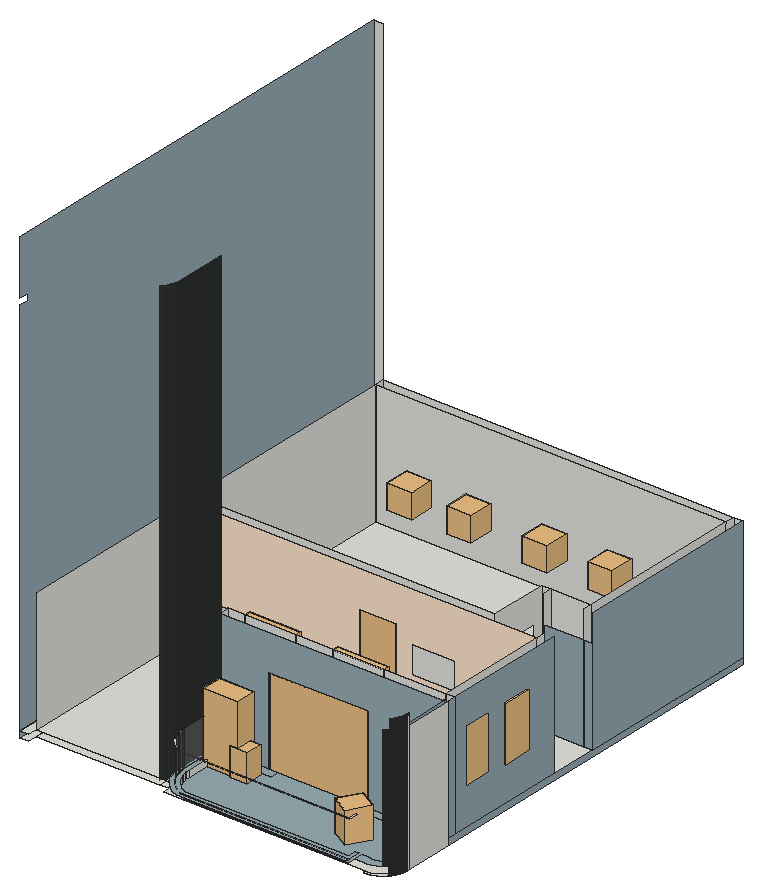
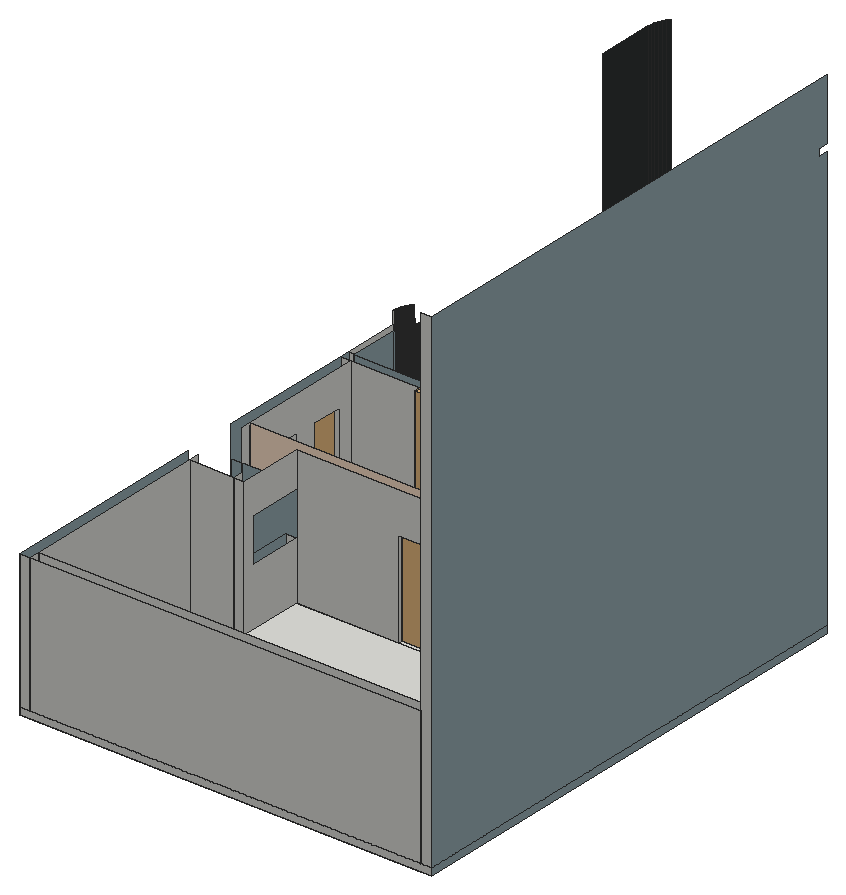
# SketchUp Ruby script. Lengths in inches.
U = 1.inch
M = Sketchup.active_model
def pt(a) = Geom::Point3d.new(a.map { |v| v * U })
def face(e, loops, mat)
  f = e.add_face(loops[0].map { |a| pt(a) })
  loops[1..].each { |l| e.add_face(l.map { |a| pt(a) }).erase! }
  f.material = f.back_material = mat if mat
  f
end
# faces: each face lists its corners as indices into pts; further lists are holes
def faces(e, pts, list, mat = nil) = list.each { |f| face(e, (f[0].is_a?(Array) ? f : [f]).map { |l| l.map { |i| pts[i] } }, mat) }
# xy, xz, yz: faces in a plane at the given z, y or x. An outline is a flat list of corners, or four numbers for a rectangle; further outlines are holes
def ring(l) = l.size == 4 ? [[l[0], l[1]], [l[2], l[1]], [l[2], l[3]], [l[0], l[3]]] : l.each_slice(2).to_a
def flat(e, list, mat, &to3) = list.each { |f| face(e, (f[0].is_a?(Array) ? f : [f]).map { |l| ring(l).map { |u, v| to3.(u, v) } }, mat) }
def xy(e, z, list, mat = nil) = flat(e, list, mat) { |x, y| [x, y, z] }
def xz(e, y, list, mat = nil) = flat(e, list, mat) { |x, z| [x, y, z] }
def yz(e, x, list, mat = nil) = flat(e, list, mat) { |y, z| [x, y, z] }
def lines(e, pts, list) = list.each { |a, b| e.add_line(pt(pts[a]), pt(pts[b])) }
# prism: a flat outline (further loops are holes) pulled along v
def prism(e, loops, v, mat = nil)
  f = face(e, loops, mat); d = Geom::Vector3d.new(v.map { |x| x * U })
  f.pushpull(f.normal.samedirection?(d) ? d.length : -d.length)
end
def box(e, o, s, mat = nil) = prism(e, [[o, [o[0] + s[0], o[1], o[2]], [o[0] + s[0], o[1] + s[1], o[2]], [o[0], o[1] + s[1], o[2]]]], [0, 0, s[2]], mat)
def at(x, y, z, deg = 0) = Geom::Transformation.translation(pt([x, y, z])) * Geom::Transformation.rotation(ORIGIN, Z_AXIS, deg.degrees)
def axes(o, x, y, z) = Geom::Transformation.new([*x, 0, *y, 0, *z, 0, *pt(o).to_a, 1])
def part(name) = M.definitions.add(name)
# library, detail: a bought-in or finely detailed component or shape, given as its bounding box
def library(name, o, s) = part(name).tap { |d| box(d.entities, o, s) }
def detail(e, o, s) = box(e.add_group.entities, o, s)
def put(e, d, t, mat = nil) = e.add_instance(d, t).tap { |i| i.material = mat if mat }
def group(e, t, mat = nil) = e.add_group.tap { |g| g.transformation = t; g.material = mat if mat }.entities
root = M.entities
M.materials.add("Generic").color = [150, 171, 178]
M.materials.add("Generic\#1").color = [47, 50, 50]
M.materials.add("Glass Thin Clear 001").color = [252, 250, 250]
M.materials["Glass Thin Clear 001"].alpha = 0.1
M.materials.add("[Color C01]").color = [255, 229, 204]
c1 = library("Chair 288 019",[-10.59,-11.4,0],[21.2,22.8,30.25])
c2 = library("Potted Plant 50-24",[-2.18,-2.1,0],[4.36,4.2,6.7])
c3 = library("Plant 260 020",[-18.86,-7.03,0.01],[33.61,20.04,67.26])
c4 = library("Window 46-47",[-61.02,-2.17,0],[122.04,4.34,74.02])
c5 = library("Curtains 003",[-24.98,-2.79,0.01],[49.96,5.58,117.31])
c6 = library("Window 46-05",[-17.86,-2.78,0],[35.72,4.26,58.96])
c7 = library("Door 243 053",[-21.6,-2.79,-0.07],[43.2,5.58,82.64])
c8 = library("Omni Light",[-12,-12,-12],[24,24,24])
xy(root,120,[[337.222,41.748,337.222,42.0625,337.846,42.071,338.474,42.095,339.101,42.136,339.726,42.194,340.35,42.268,340.972,42.358,341.591,42.464,342.207,42.587,342.82,42.726,343.429,42.88,344.034,43.051,344.634,43.237,345.229,43.439,345.818,43.657,346.402,43.889,346.979,44.137,347.55,44.4,348.113,44.678,348.669,44.971,349.218,45.278,349.758,45.599,350.289,45.934,350.811,46.283,351.324,46.646,351.828,47.022,352.321,47.411,352.804,47.813,353.277,48.227,353.738,48.654,354.188,49.092,354.627,49.542,355.053,50.003,355.467,50.476,355.869,50.959,356.258,51.452,356.634,51.956,356.997,52.469,357.346,52.991,357.681,53.523,358.002,54.0625,358.309,54.611,358.602,55.167,358.88,55.73,359.143,56.301,359.391,56.878,359.624,57.462,359.841,58.051,360.043,58.646,360.229,59.246,360.4,59.851,360.554,60.46,360.693,61.073,360.816,61.689,360.922,62.308,361.012,62.93,361.086,63.554,361.144,64.179,361.185,64.806,361.209,65.434,361.218,66.0625,361.532,66.058,361.523,65.426,361.498,64.79,361.457,64.155,361.399,63.521,361.324,62.889,361.232,62.259,361.125,61.632,361,61.007,360.86,60.386,360.703,59.77,360.531,59.157,360.342,58.549,360.137,57.946,359.917,57.349,359.681,56.758,359.43,56.173,359.163,55.595,358.882,55.024,358.585,54.461,358.274,53.905,357.949,53.358,357.609,52.82,357.256,52.291,356.888,51.771,356.507,51.261,356.113,50.761,355.706,50.272,355.287,49.793,354.854,49.326,354.41,48.87,353.954,48.426,353.487,47.994,353.008,47.574,352.519,47.167,352.019,46.773,351.509,46.392,350.989,46.025,350.46,45.671,349.922,45.331,349.375,45.006,348.819,44.695,348.256,44.398,347.685,44.117,347.107,43.85,346.522,43.599,345.931,43.363,345.334,43.143,344.731,42.938,344.123,42.75,343.511,42.577,342.894,42.42,342.273,42.28,341.648,42.155,341.021,42.048,340.391,41.956,339.759,41.882,339.125,41.823,338.49,41.782,337.854,41.757],[1.218,42.0625,10.218,474.0625],[337.218,42.0625,337.184,44.654,337.778,44.662,338.338,44.684,338.897,44.72,339.455,44.772,340.012,44.838,340.567,44.918,341.119,45.013,341.669,45.122,342.215,45.246,342.758,45.384,343.298,45.536,343.833,45.702,344.364,45.882,344.89,46.076,345.41,46.284,345.925,46.505,346.434,46.74,346.937,46.988,347.433,47.249,347.922,47.523,348.403,47.809,348.877,48.108,349.343,48.42,349.801,48.743,350.25,49.078,350.69,49.425,351.121,49.784,351.542,50.153,351.954,50.534,352.355,50.925,352.746,51.326,353.127,51.738,353.496,52.159,353.855,52.59,354.202,53.03,354.537,53.479,354.861,53.937,355.172,54.403,355.471,54.877,355.757,55.358,356.031,55.847,356.292,56.343,356.54,56.846,356.775,57.355,356.996,57.87,357.204,58.391,357.398,58.916,357.578,59.447,357.744,59.982,357.896,60.522,358.034,61.065,358.158,61.612,358.267,62.161,358.362,62.714,358.442,63.268,358.508,63.825,358.56,64.383,358.596,64.942,358.618,65.502,358.626,66.096,361.218,66.0625,361.209,65.434,361.185,64.806,361.144,64.179,361.086,63.554,361.012,62.93,360.922,62.308,360.816,61.689,360.693,61.073,360.554,60.46,360.4,59.851,360.229,59.246,360.043,58.646,359.841,58.051,359.624,57.462,359.391,56.878,359.143,56.301,358.88,55.73,358.602,55.167,358.309,54.611,358.002,54.0625,357.681,53.523,357.346,52.991,356.997,52.469,356.634,51.956,356.258,51.452,355.869,50.959,355.467,50.476,355.053,50.003,354.627,49.542,354.188,49.092,353.738,48.654,353.277,48.227,352.804,47.813,352.321,47.411,351.828,47.022,351.324,46.646,350.811,46.283,350.289,45.934,349.758,45.599,349.218,45.278,348.669,44.971,348.113,44.678,347.55,44.4,346.979,44.137,346.402,43.889,345.818,43.657,345.229,43.439,344.634,43.237,344.034,43.051,343.429,42.88,342.82,42.726,342.207,42.587,341.591,42.464,340.972,42.358,340.35,42.268,339.726,42.194,339.101,42.136,338.474,42.095,337.846,42.071,337.222,42.0625],[[139.218,44.654,139.218,171.0625,361.218,171.0625,361.218,66.0625,358.626,66.096,358.618,65.502,358.596,64.942,358.56,64.383,358.508,63.825,358.442,63.268,358.362,62.714,358.267,62.161,358.158,61.612,358.034,61.065,357.896,60.522,357.744,59.982,357.578,59.447,357.398,58.916,357.204,58.391,356.996,57.87,356.775,57.355,356.54,56.846,356.292,56.343,356.031,55.847,355.757,55.358,355.471,54.877,355.172,54.403,354.861,53.937,354.537,53.479,354.202,53.03,353.855,52.59,353.496,52.159,353.127,51.738,352.746,51.326,352.355,50.925,351.954,50.534,351.542,50.153,351.121,49.784,350.69,49.425,350.25,49.078,349.801,48.743,349.343,48.42,348.877,48.108,348.403,47.809,347.922,47.523,347.433,47.249,346.937,46.988,346.434,46.74,345.925,46.505,345.41,46.284,344.89,46.076,344.364,45.882,343.833,45.702,343.298,45.536,342.758,45.384,342.215,45.246,341.669,45.122,341.119,45.013,340.567,44.918,340.012,44.838,339.455,44.772,338.897,44.72,338.338,44.684,337.778,44.662,337.184,44.654],[302.424,124.131,314.611,143.851],[194.174,124.131,206.361,143.851]],[10.218,51.0625,10.218,465.0625,352.218,465.0625,352.218,180.0625,130.218,180.0625,130.218,51.0625],
  [130.218,51.0625,130.218,180.0625,352.218,180.0625,352.218,171.0625,139.218,171.0625,139.218,51.0625],[130.218,51.0625,139.218,171.0625],[130.218,171.0625,352.218,180.0625],[352.218,171.0625,361.218,465.0625],[10.218,465.0625,361.218,474.0625]])
xy(root,126,[[1.218,42.0625,10.218,474.0625],[10.218,51.0625,130.218,51.0625,130.218,123.0625,352.218,123.0625,352.218,234.0625,215.03,234.0625,215.03,243.0625,179.03,243.0625,179.03,234.0625,10.218,234.0625],[130.218,51.0625,139.218,123.0625],[139.218,114.0625,187.218,123.0625],[283.218,114.0625,361.218,123.0625],
  [352.218,123.0625,361.218,243.0625],[10.218,234.0625,179.03,243.0625],[215.03,234.0625,352.218,243.0625],[10.218,243.0625,304.218,243.0625,304.218,300.0625,352.218,300.0625,352.218,465.0625,10.218,465.0625],[304.218,243.0625,313.218,300.0625],
  [313.218,243.0625,361.218,291.0625],[313.218,291.0625,352.218,300.0625],[352.218,291.0625,361.218,474.0625],[10.218,465.0625,352.218,474.0625]])
xy(root,126,[[165.323,38.075,325.076,38.075,325.076,54.944,334.449,54.128,334.855,54.104,335.261,54.093,335.668,54.094,336.074,54.107,336.48,54.131,336.884,54.168,337.288,54.217,337.69,54.278,338.09,54.35,338.488,54.434,338.883,54.53,339.275,54.638,339.663,54.757,340.048,54.888,340.429,55.03,340.806,55.183,341.178,55.347,341.545,55.522,341.906,55.708,342.262,55.905,342.612,56.111,342.956,56.329,343.293,56.556,343.623,56.793,343.946,57.04,344.262,57.296,344.569,57.561,344.869,57.836,345.161,58.119,345.444,58.411,345.719,58.711,345.984,59.019,346.24,59.334,346.487,59.657,346.724,59.987,346.951,60.324,347.169,60.668,347.376,61.018,347.572,61.374,347.758,61.735,347.933,62.102,348.097,62.474,348.25,62.851,348.392,63.232,348.523,63.617,348.642,64.005,348.75,64.397,348.846,64.792,348.93,65.19,349.003,65.59,349.063,65.992,349.112,66.396,349.149,66.8,349.173,67.206,349.186,67.613,349.187,68.019,349.176,68.425,349.152,68.831,349.076,69.709,349.076,105.921,275.076,105.921,275.076,114.921,195.359,114.921,195.359,105.921,147.359,105.921,147.359,65.284,147.52,62.113,147.969,59.178,148.712,56.303,149.743,53.518,151.049,50.852,152.618,48.331,154.434,45.982,156.478,43.828,158.729,41.892,161.164,40.193,163.759,38.749],[335.156,45.951,335.803,45.953,336.45,45.973,337.096,46.012,337.741,46.071,338.383,46.148,339.023,46.245,339.66,46.36,340.293,46.495,340.922,46.647,341.546,46.819,342.165,47.009,342.778,47.216,343.385,47.442,343.984,47.686,344.576,47.948,345.161,48.227,345.736,48.523,346.303,48.835,346.86,49.165,347.407,49.511,347.944,49.873,348.47,50.25,348.984,50.643,349.486,51.051,349.977,51.474,350.454,51.911,350.919,52.361,351.37,52.826,351.806,53.303,352.229,53.794,352.637,54.296,353.03,54.811,353.408,55.336,353.769,55.873,354.115,56.42,354.445,56.977,354.758,57.544,355.054,58.119,355.332,58.704,355.594,59.296,355.838,59.895,356.064,60.502,356.272,61.115,356.461,61.734,356.633,62.358,356.786,62.987,356.92,63.62,357.035,64.257,357.132,64.897,357.209,65.54,357.268,66.184,357.307,66.83,357.328,67.477,357.329,68.124,357.311,68.771,357.274,69.418,357.218,70.0625,357.218,114.0625,349.076,105.921,349.076,69.709,349.152,68.831,349.176,68.425,349.187,68.019,349.186,67.613,349.173,67.206,349.149,66.8,349.112,66.396,349.063,65.992,349.003,65.59,348.93,65.19,348.846,64.792,348.75,64.397,348.642,64.005,348.523,63.617,348.392,63.232,348.25,62.851,348.097,62.474,347.933,62.102,347.758,61.735,347.572,61.374,347.376,61.018,347.169,60.668,346.951,60.324,346.724,59.987,346.487,59.657,346.24,59.334,345.984,59.019,345.719,58.711,345.444,58.411,345.161,58.119,344.869,57.836,344.569,57.561,344.262,57.296,343.946,57.04,343.623,56.793,343.293,56.556,342.956,56.329,342.612,56.111,342.262,55.905,341.906,55.708,341.545,55.522,341.178,55.347,340.806,55.183,340.429,55.03,340.048,54.888,339.663,54.757,339.275,54.638,338.883,54.53,338.488,54.434,338.09,54.35,337.69,54.278,337.288,54.217,336.884,54.168,336.48,54.131,336.074,54.107,335.668,54.094,335.261,54.093,334.855,54.104,334.449,54.128,325.076,54.944,325.076,46.0625,333.218,46.0625,333.862,46.006,334.509,45.969],[147.359,105.921,195.359,105.921,195.359,114.921,275.076,114.921,275.076,105.921,349.076,105.921,357.218,114.0625,283.218,114.0625,283.218,123.0625,187.218,123.0625,187.218,114.0625,139.218,114.0625]],"Generic")
xy(root,132,[[163.644,29.933,328.648,29.933,328.648,33.506,164.381,33.506,161.739,34.644,158.74,36.313,155.925,38.277,153.323,40.515,150.96,43.004,148.861,45.72,147.048,48.634,145.538,51.716,144.347,54.935,143.487,58.258,142.968,61.651,142.79,65.169,142.79,105.438,143.787,104.441,143.787,65.194,143.961,61.751,144.465,58.459,145.299,55.233,146.455,52.109,147.92,49.118,149.681,46.29,151.718,43.654,154.011,41.237,156.536,39.065,159.269,37.159,162.179,35.539,164.586,34.503,328.648,34.503,328.648,46.0625,325.076,46.0625,325.076,38.075,165.323,38.075,163.759,38.749,161.164,40.193,158.729,41.892,156.478,43.828,154.434,45.982,152.618,48.331,151.049,50.852,149.743,53.518,148.712,56.303,147.969,59.178,147.52,62.113,147.359,65.284,147.359,105.921,139.218,114.0625,139.218,65.078,139.41,61.289,139.983,57.539,140.933,53.865,142.25,50.307,143.919,46.9,145.924,43.678,148.244,40.676,150.856,37.924,153.732,35.45,156.844,33.279,160.159,31.434]],"Generic")
xy(root,162.223,[[352.218,136.159,361.218,164.284],[352.218,182.159,361.218,210.284]])
xy(root,168,[[164.381,33.506,161.739,34.644,158.74,36.313,155.925,38.277,153.323,40.515,150.96,43.004,148.861,45.72,147.048,48.634,145.538,51.716,144.347,54.935,143.487,58.258,142.968,61.651,142.79,65.169,142.79,105.438,143.787,104.441,143.787,65.194,143.961,61.751,144.465,58.459,145.299,55.233,146.455,52.109,147.92,49.118,149.681,46.29,151.718,43.654,154.011,41.237,156.536,39.065,159.269,37.159,162.179,35.539,164.586,34.503,328.648,34.503,328.648,42.0625,329.645,42.0625,329.645,33.506]])
xz(root,114.0625,[[357.218,126,361.218,246]])
xz(root,114.0625,[[139.218,126,187.218,126,187.218,210,283.218,210,283.218,126,357.218,126,357.218,245,139.218,245]],"Generic")
xz(root,123.0625,[[130.218,126,139.218,245],[139.218,126,139.218,246,352.218,246,352.218,126,283.218,126,283.218,210,187.218,210,187.218,126],[352.218,126,361.218,246]])
xz(root,136.159,[[352.218,162.223,361.218,215.411]])
xz(root,164.284,[[352.218,162.223,361.218,215.411]])
xz(root,182.159,[[352.218,162.223,361.218,215.411]])
xz(root,210.284,[[352.218,162.223,361.218,215.411]])
xz(root,234.0625,[[[10.218,126,179.03,126,179.03,210,215.03,210,215.03,126,352.218,126,352.218,246,10.218,246],[230.012,170.836,272.45,198.024]]],"[Color C01]")
xz(root,243.0625,[[10.218,126,10.218,246,304.218,246,304.218,126,215.03,126,215.03,210,179.03,210,179.03,126],[304.218,126,313.218,177.1]])
xz(root,243.0625,[[313.218,126,313.218,177.1,304.218,177.1,304.218,215.248,313.218,215.248,313.218,219.122,352.218,219.122,352.218,126],[352.218,126,361.218,219.122]],"Generic")
xz(root,291.0625,[[313.218,126,352.218,219.122],[352.218,126,361.218,219.122]],"Generic")
xz(root,300.0625,[[304.218,126,313.218,246],[313.218,126,352.218,246]])
xz(root,465.0625,[[10.218,126,352.218,246]])
xz(root,474.0625,[[1.218,120,361.218,126],[1.218,126,10.218,558],[10.218,126,352.218,246],[352.218,126,361.218,246]])
yz(root,1.218,[[42.0625,120,474.0625,126],[42.0625,126,42.0625,498,51.0625,498,51.0625,504.044,42.0625,504.044,42.0625,558,474.0625,558,474.0625,126]],"Generic")
yz(root,10.218,[[51.0625,126,234.0625,246],[234.0625,126,243.0625,246],[243.0625,126,465.0625,246],[465.0625,126,474.0625,246]])
yz(root,130.218,[[51.0625,126,123.0625,245]])
yz(root,139.218,[[51.0625,126,65.078,126.3125],[65.078,126,114.0625,132],[114.0625,126,123.0625,245]])
yz(root,139.218,[[65.078,132,114.0625,558]],"Generic\#1")
yz(root,142.412,[[65.159,168,106.351,168.5625]])
yz(root,142.79,[[65.169,168,104.028,168.5625]])
yz(root,142.79,[[65.169,132,105.438,168]],"Glass Thin Clear 001")
yz(root,143.787,[[65.194,168,103.032,168.5625]])
yz(root,143.787,[[65.194,132,104.441,168]],"Glass Thin Clear 001")
yz(root,144.165,[[65.204,168,104.598,168.5625]])
yz(root,147.359,[[65.284,126,105.921,132]])
yz(root,179.03,[[234.0625,126,243.0625,210]])
yz(root,187.218,[[114.0625,126,123.0625,210]])
yz(root,215.03,[[234.0625,126,243.0625,210]])
yz(root,283.218,[[114.0625,126,123.0625,210]])
yz(root,304.218,[[243.0625,126,243.0625,177.1,291.0625,177.1,291.0625,215.248,243.0625,215.248,243.0625,246,300.0625,246,300.0625,126]])
yz(root,313.218,[[291.0625,126,300.0625,246]])
yz(root,313.218,[[243.0625,126,291.0625,177.1]],"Generic")
yz(root,352.218,[[[123.0625,126,234.0625,246],[136.159,162.223,164.284,215.411],[182.159,162.223,210.284,215.411]],[234.0625,126,243.0625,246],[291.0625,126,300.0625,246],[300.0625,126,465.0625,246],[465.0625,126,474.0625,246]])
yz(root,357.218,[[70.0625,126,114.0625,245]],"Generic")
yz(root,361.218,[[66.0625,120,114.0625,246]])
yz(root,361.218,[[114.0625,120,474.0625,126],[114.0625,126,123.0625,246],[[123.0625,126,243.0625,246],[136.159,162.223,164.284,215.411],[182.159,162.223,210.284,215.411]],[291.0625,126,474.0625,246]],"Generic")
p = [[355.053,50.003,120],[355.467,50.476,120],[355.467,50.476,246],[355.053,50.003,246],[356.113,50.761,120],[355.706,50.272,120],
  [355.706,50.272,257],[356.113,50.761,257],[355.869,50.959,120],[355.869,50.959,246],[356.507,51.261,120],[356.507,51.261,257],
  [356.258,51.452,120],[356.258,51.452,246],[356.888,51.771,120],[356.888,51.771,257],[356.634,51.956,120],[356.634,51.956,246],
  [357.256,52.291,120],[357.256,52.291,257],[356.997,52.469,120],[356.997,52.469,246],[357.609,52.82,120],[357.609,52.82,257],
  [357.346,52.991,120],[357.346,52.991,246],[357.949,53.358,120],[357.949,53.358,257],[357.681,53.523,120],[357.681,53.523,246],
  [358.274,53.905,120],[358.274,53.905,257],[358.002,54.0625,120],[358.002,54.0625,246],[358.585,54.461,120],[358.585,54.461,257],
  [358.309,54.611,120],[358.309,54.611,246],[358.882,55.024,120],[358.882,55.024,257],[358.602,55.167,120],[358.602,55.167,246],
  [359.163,55.595,120],[359.163,55.595,257],[358.88,55.73,120],[358.88,55.73,246],[359.43,56.173,120],[359.43,56.173,257],
  [359.143,56.301,120],[359.143,56.301,246],[359.681,56.758,120],[359.681,56.758,257],[359.391,56.878,120],[359.391,56.878,246],
  [359.917,57.349,120],[359.917,57.349,257],[359.624,57.462,120],[359.624,57.462,246],[360.137,57.946,120],[360.137,57.946,257],
  [359.841,58.051,120],[359.841,58.051,246],[360.342,58.549,120],[360.342,58.549,257],[360.043,58.646,120],[360.043,58.646,246],
  [360.531,59.157,120],[360.531,59.157,257],[360.229,59.246,120],[360.229,59.246,246],[360.4,59.851,120],[360.4,59.851,246],
  [360.703,59.77,120],[360.703,59.77,257],[360.86,60.386,120],[360.86,60.386,257],[360.554,60.46,120],[360.554,60.46,246],
  [361,61.007,120],[361,61.007,257],[360.693,61.073,120],[360.693,61.073,246],[361.125,61.632,120],[361.125,61.632,257],
  [360.816,61.689,120],[360.816,61.689,246],[361.232,62.259,120],[361.232,62.259,257],[360.922,62.308,120],[360.922,62.308,246],
  [361.012,62.93,120],[361.012,62.93,246],[361.324,62.889,120],[361.324,62.889,257],[361.086,63.554,120],[361.086,63.554,246],
  [361.399,63.521,120],[361.399,63.521,257],[361.457,64.155,120],[361.457,64.155,257],[361.144,64.179,120],[361.144,64.179,246],
  [361.094,63.642,246],[361.185,64.806,120],[361.185,64.806,246],[361.498,64.79,120],[361.498,64.79,257],[361.209,65.434,120],
  [361.209,65.434,246],[361.523,65.426,120],[361.523,65.426,257],[361.218,66.0625,120],[361.218,66.0625,246],[361.532,66.058,120],
  [361.532,66.058,257],[361.218,66.0625,257],[361.218,66.0625,252],[140.933,53.865,126],[142.25,50.307,126],[142.25,50.307,132],
  [140.933,53.865,132],[348.984,50.643,126],[348.47,50.25,126],[348.47,50.25,245],[348.984,50.643,245],[349.486,51.051,126],
  [349.486,51.051,245],[151.049,50.852,126],[149.743,53.518,126],[149.743,53.518,132],[151.049,50.852,132],[349.977,51.474,126],
  [349.977,51.474,245],[350.454,51.911,126],[350.454,51.911,245],[350.919,52.361,126],[350.919,52.361,245],[351.37,52.826,126],
  [351.37,52.826,245],[351.806,53.303,126],[351.806,53.303,245],[352.229,53.794,126],[352.229,53.794,245],[148.712,56.303,126],
  [148.712,56.303,132],[352.637,54.296,126],[352.637,54.296,245],[139.983,57.539,126],[139.983,57.539,132],[353.03,54.811,126],
  [353.03,54.811,245],[353.408,55.336,126],[353.408,55.336,245],[353.769,55.873,126],[353.769,55.873,245],[354.115,56.42,126],
  [354.115,56.42,245],[147.969,59.178,126],[147.969,59.178,132],[354.445,56.977,126],[354.445,56.977,245],[354.758,57.544,126],
  [354.758,57.544,245],[139.41,61.289,126],[139.41,61.289,132],[355.054,58.119,126],[355.054,58.119,245],[355.332,58.704,126],
  [355.332,58.704,245],[355.594,59.296,126],[355.594,59.296,245],[147.52,62.113,126],[147.52,62.113,132],[355.838,59.895,126],
  [355.838,59.895,245],[356.064,60.502,126],[356.064,60.502,245],[356.272,61.115,126],[356.272,61.115,245],[356.461,61.734,126],
  [356.461,61.734,245],[139.218,65.078,126],[139.218,65.078,132],[139.218,65.078,126.3125],[356.633,62.358,126],[356.633,62.358,245],
  [147.359,65.284,126],[147.359,65.284,132],[356.786,62.987,126],[356.786,62.987,245],[356.92,63.62,126],[356.92,63.62,245],
  [357.035,64.257,126],[357.035,64.257,245],[357.132,64.897,126],[357.132,64.897,245],[357.209,65.54,126],[357.209,65.54,245],
  [357.268,66.184,126],[357.268,66.184,245],[357.307,66.83,126],[357.307,66.83,245],[357.328,67.477,126],[357.328,67.477,245],
  [357.329,68.124,126],[357.329,68.124,245],[357.311,68.771,126],[357.311,68.771,245],[357.274,69.418,126],[357.274,69.418,245],
  [357.218,70.0625,126],[357.218,70.0625,245],[147.359,105.921,126],[139.218,114.0625,126],[139.218,114.0625,132],[147.359,105.921,132],
  [134.457,51.0625,504.044],[134.457,51.0625,558],[132.476,48.804,558],[132.476,48.804,126.3125],[134.457,51.0625,126.3125],[134.457,51.0625,498],
  [134.461,51.067,126.3125],[134.461,51.067,558],[136.134,53.57,126.3125],[136.134,53.57,558],[137.466,56.271,126.3125],[137.466,56.271,558],
  [138.433,59.121,126.3125],[138.433,59.121,558],[139.021,62.074,126.3125],[139.021,62.074,558],[139.218,65.078,390],[139.218,65.078,558],
  [139.218,65.078,245],[139.218,65.078,246],[139.218,65.078,252],[139.218,65.078,257],[139.218,65.078,362],[139.218,65.078,378],
  [147.92,49.118,132],[146.455,52.109,132],[146.455,52.109,168],[147.92,49.118,168],[144.347,54.935,132],[145.538,51.716,132],
  [145.538,51.716,168],[144.347,54.935,168],[145.299,55.233,132],[145.299,55.233,168],[143.487,58.258,132],[143.487,58.258,168],
  [144.465,58.459,132],[144.465,58.459,168],[142.968,61.651,132],[142.968,61.651,168],[143.961,61.751,132],[143.961,61.751,168],
  [142.79,65.169,132],[142.79,65.169,168],[143.787,65.194,132],[143.787,65.194,168],[143.787,104.441,132],[142.79,105.438,132],
  [142.79,105.438,168],[143.787,104.441,168],[147.92,49.118,168.5625],[146.455,52.109,168.5625],[146.803,52.258,168],[146.803,52.258,168.5625],
  [148.252,49.301,168.5625],[148.252,49.301,168],[145.189,51.567,168],[145.189,51.567,168.5625],[143.985,54.822,168.5625],[143.985,54.822,168],
  [144.347,54.935,168.5625],[145.538,51.716,168.5625],[145.299,55.233,168.5625],[145.661,55.347,168],[145.661,55.347,168.5625],[143.116,58.182,168.5625],
  [143.116,58.182,168],[143.487,58.258,168.5625],[144.465,58.459,168.5625],[144.836,58.535,168],[144.836,58.535,168.5625],[142.591,61.612,168.5625],
  [142.591,61.612,168],[142.968,61.651,168.5625],[143.961,61.751,168.5625],[144.338,61.79,168],[144.338,61.79,168.5625],[142.412,65.159,168.5625],
  [142.412,65.159,168],[142.79,65.169,168.5625],[143.787,65.194,168.5625],[144.165,65.204,168],[144.165,65.204,168.5625],[142.412,106.351,168],
  [142.412,106.351,168.5625],[144.165,104.598,168.5625],[144.165,104.598,168],[354.182,49.098,120.064],[356.252,51.457,120.062],[357.996,54.067,120.056],
  [359.385,56.881,120.047],[360.396,59.853,120.035],[361.01,62.931,120.019]]
faces(root,p,[[0,1,2,3],[4,5,6,7],[1,8,9,2],[10,4,7,11],[8,12,13,9],[14,10,11,15],[12,16,17,13],[18,14,15,19],
  [16,20,21,17],[22,18,19,23],[20,24,25,21],[26,22,23,27],[24,28,29,25],[30,26,27,31],[28,32,33,29],[34,30,31,35],
  [32,36,37,33],[38,34,35,39],[36,40,41,37],[42,38,39,43],[40,44,45,41],[46,42,43,47],[44,48,49,45],[50,46,47,51],
  [48,52,53,49],[54,50,51,55],[52,56,57,53],[58,54,55,59],[56,60,61,57],[62,58,59,63],[60,64,65,61],[66,62,63,67],
  [64,68,69,65],[68,70,71,69],[72,66,67,73],[74,72,73,75],[70,76,77,71],[78,74,75,79],[76,80,81,77],[82,78,79,83],
  [80,84,85,81],[86,82,83,87],[84,88,89,85],[88,90,91,89],[92,86,87,93],[90,94,95,91],[96,92,93,97],[98,96,97,99],
  [94,100,101,102,95],[100,103,104,101],[105,98,99,106],[103,107,108,104],[109,105,106,110],[107,111,112,108],[113,109,110,114],[111,113,114,115,116,112],
  [127,128,129,130],[128,143,144,129],[143,157,158,144],[157,171,172,158],[171,186,187,172],[212,213,214,215],[262,263,264,265],[266,243,242,267],
  [268,269,270,271],[272,273,274,275],[276,247,246,277],[267,242,249,278],[279,280,269,268],[275,274,281,282],[283,251,247,276],[278,249,253,284],
  [285,286,280,279],[282,281,287,288],[289,255,251,283],[284,253,257,290],[291,292,286,285],[288,287,293,294],[295,259,255,289],[290,257,261,296],
  [297,298,292,291],[299,300,301,302]])
faces(root,p,[[117,118,119,120],[121,122,123,124],[125,121,124,126],[131,125,126,132],[133,131,132,134],[135,133,134,136],[137,135,136,138],[139,137,138,140],
  [141,139,140,142],[145,141,142,146],[147,117,120,148],[149,145,146,150],[151,149,150,152],[153,151,152,154],[155,153,154,156],[159,155,156,160],
  [161,159,160,162],[163,147,148,164],[165,161,162,166],[167,165,166,168],[169,167,168,170],[173,169,170,174],[175,173,174,176],[177,175,176,178],
  [179,177,178,180],[181,163,164,182,183],[184,179,180,185],[188,184,185,189],[190,188,189,191],[192,190,191,193],[194,192,193,195],[196,194,195,197],
  [198,196,197,199],[200,198,199,201],[202,200,201,203],[204,202,203,205],[206,204,205,207],[208,206,207,209],[210,208,209,211]],"Generic")
faces(root,p,[[216,217,218,219,220,221],[222,223,217,216,221,220],[224,225,223,222],[226,227,225,224],[228,229,227,226],[230,231,229,228],[232,233,231,230,183,182,234,235,236,237,238,239]],"Generic\#1")
faces(root,p,[[240,241,242,243],[244,245,246,247],[241,248,249,242],[250,244,247,251],[248,252,253,249],[254,250,251,255],[252,256,257,253],[258,254,255,259],
  [256,260,261,257]],"Glass Thin Clear 001")
lines(root,p,[[303,304],[304,305],[305,306],[306,307],[307,308],[308,111]])
put(root,c1,at(302.55,72.57,126,-30))
put(root,c2,axes([179.53,94.01,126],[4,0,0],[0,4,0],[0,0,4]))
put(root,c3,at(162.66,94.23,126))
put(root,c4,axes([234.92,116.21,125.95],[0.79167,0,0],[0,1,0],[0,0,1.14]))
put(root,c5,at(267.15,125.86,128.68))
put(root,c5,at(181.09,125.86,128.68))
put(root,c6,axes([358.39,149.9,162.22],[0,0.80542,0],[-0.8,0,0],[0,0,0.90212]))
put(root,c6,axes([360.98,196.22,162.16],[0,0.78717,0],[-1,0,0],[0,0,0.90321]))
put(root,c7,axes([197.03,236.85,126],[0.83329,0,0],[0,1,0],[0,0,1.01736]))
put(root,c8,at(114.47,448.09,172.75))
put(root,c8,at(188.35,448.09,172.75))
put(root,c8,at(56.1,448.09,172.75))
put(root,c8,at(251.97,448.09,172.75))
